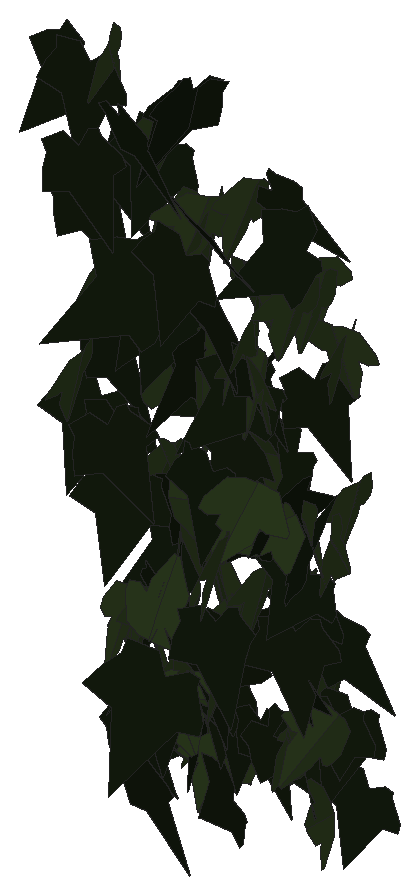
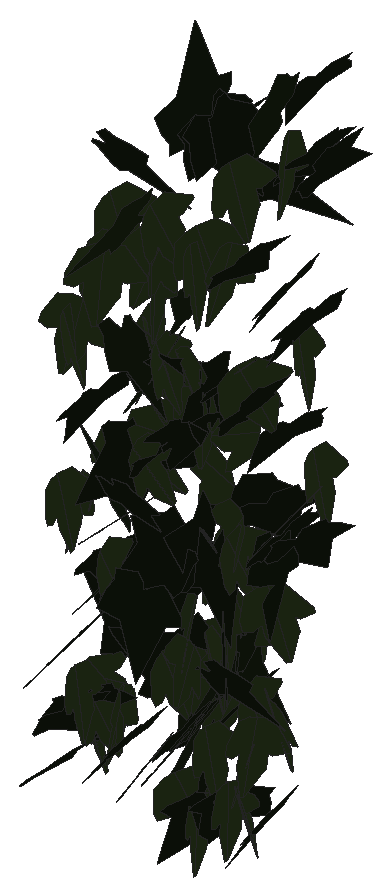
# SketchUp Ruby script. Lengths in inches.
U = 1.inch
M = Sketchup.active_model
def pt(a) = Geom::Point3d.new(a.map { |v| v * U })
def face(e, loops, mat)
  f = e.add_face(loops[0].map { |a| pt(a) })
  loops[1..].each { |l| e.add_face(l.map { |a| pt(a) }).erase! }
  f.material = f.back_material = mat if mat
  f
end
# faces: each face lists its corners as indices into pts; further lists are holes
def faces(e, pts, list, mat = nil) = list.each { |f| face(e, (f[0].is_a?(Array) ? f : [f]).map { |l| l.map { |i| pts[i] } }, mat) }
# xy, xz, yz: faces in a plane at the given z, y or x. An outline is a flat list of corners, or four numbers for a rectangle; further outlines are holes
def ring(l) = l.size == 4 ? [[l[0], l[1]], [l[2], l[1]], [l[2], l[3]], [l[0], l[3]]] : l.each_slice(2).to_a
def flat(e, list, mat, &to3) = list.each { |f| face(e, (f[0].is_a?(Array) ? f : [f]).map { |l| ring(l).map { |u, v| to3.(u, v) } }, mat) }
def xy(e, z, list, mat = nil) = flat(e, list, mat) { |x, y| [x, y, z] }
def xz(e, y, list, mat = nil) = flat(e, list, mat) { |x, z| [x, y, z] }
def yz(e, x, list, mat = nil) = flat(e, list, mat) { |y, z| [x, y, z] }
def lines(e, pts, list) = list.each { |a, b| e.add_line(pt(pts[a]), pt(pts[b])) }
# prism: a flat outline (further loops are holes) pulled along v
def prism(e, loops, v, mat = nil)
  f = face(e, loops, mat); d = Geom::Vector3d.new(v.map { |x| x * U })
  f.pushpull(f.normal.samedirection?(d) ? d.length : -d.length)
end
def box(e, o, s, mat = nil) = prism(e, [[o, [o[0] + s[0], o[1], o[2]], [o[0] + s[0], o[1] + s[1], o[2]], [o[0], o[1] + s[1], o[2]]]], [0, 0, s[2]], mat)
def at(x, y, z, deg = 0) = Geom::Transformation.translation(pt([x, y, z])) * Geom::Transformation.rotation(ORIGIN, Z_AXIS, deg.degrees)
def axes(o, x, y, z) = Geom::Transformation.new([*x, 0, *y, 0, *z, 0, *pt(o).to_a, 1])
def part(name) = M.definitions.add(name)
# library, detail: a bought-in or finely detailed component or shape, given as its bounding box
def library(name, o, s) = part(name).tap { |d| box(d.entities, o, s) }
def detail(e, o, s) = box(e.add_group.entities, o, s)
def put(e, d, t, mat = nil) = e.add_instance(d, t).tap { |i| i.material = mat if mat }
def group(e, t, mat = nil) = e.add_group.tap { |g| g.transformation = t; g.material = mat if mat }.entities
root = M.entities
M.materials.add("efeu1").color = [18, 25, 13]
M.materials.add("efeu2").color = [43, 57, 29]
c1 = part("ivyleaf_9")
p = [[1.54,2.16,1.25],[1.36,2.04,1.19],[-0.21,0.99,0.68],[-0.71,1.11,0.82],[-0.85,0.86,0.67],[-0.8,0.17,0.21],
  [-0.9,-0.01,0.1],[-0.67,-0.16,-0.02],[-0.08,-0.08,-0.05],[-0.03,-0.6,-0.4],[0.65,-0.88,-0.66],[0.83,-0.6,-0.49],
  [1.29,-0.42,-0.43],[1.8125,-0.07,-0.26],[1.21,0.44,0.15]]
faces(c1.entities,p,[[0,1,2,3,4,5,6,7,8,9,10,11,12,13,14]],"efeu1")
c2 = part("ivyleaf_10")
p = [[0,0.5,-0.03],[-0.0625,2.02,-0.43],[-0.19,2.01,-0.46],[-0.54,1.05,-0.29],[-0.52,0.625,-0.18],[-0.83,0.76,-0.28],
  [-1.16,0.64,-0.33],[-1.15,0.33,-0.24],[-0.77,-0.39,0.02],[-0.3,-0.51,0.16],[0.04,-0.48,0.23],[-0.02,2.01,-0.4375],
  [-0.06,2.01,-0.43],[0.04,-0.49,0.23],[0.67,-0.49,0.14],[1.38,0.36,-0.2],[1.375,0.51,-0.24],[0.81,0.65,-0.19],
  [0.62,0.59,-0.15],[0.6,1.09,-0.28],[0.5,1.23,-0.31]]
faces(c2.entities,p,[[0,1,2,3,4,5,6,7,8,9,10],[11,12,0,13,14,15,16,17,18,19,20]],"efeu2")
put(root,c1,axes([550.52,126.8,290.29],[0.5719,-0.99368,-0.26786],[-0.00484,0.30384,-1.13749],[1.02914,0.55363,0.1435]))
put(root,c1,axes([551.15,125.6875,288.58],[-0.4997,-1.07408,0.06515],[-0.00721,-0.06848,-1.18442],[1.07603,-0.49925,0.02231]))
put(root,c2,axes([551.51,124.1,290.82],[0.18064,-1.20547,-0.05667],[-0.00234,0.05695,-1.21892],[1.2068,0.18055,0.00612]))
put(root,c2,axes([551.94,126.33,285.9375],[-1.04432,-0.39407,0.41704],[-0.30298,-0.35673,-1.0958],[0.48725,-1.06643,0.21245]))
put(root,c1,axes([551.4,124.52,297.51],[0.44186,-1.01629,-0.53112],[-0.03486,0.55702,-1.09484],[1.14617,0.40873,0.17145]))
put(root,c1,axes([551.97,123.53,302.78],[-0.34838,-0.90881,0.76609],[-0.28525,-0.71107,-0.97325],[1.15389,-0.45017,-0.00929]))
put(root,c2,axes([552.04,127.11,280.74],[-0.36388,-1.02386,-0.3654],[0.14113,0.33758,-1.08643],[1.07791,-0.38983,0.0189]))
put(root,c1,axes([552.49,125.39,287.5625],[0.62271,0.33075,-0.97016],[-1.01556,0.04545,-0.63636],[-0.13873,1.15192,0.30367]))
put(root,c2,axes([552.21,125.68,280.95],[0.98533,-0.69641,-0.01824],[-0.02055,0.00252,-1.20655],[0.69634,0.98549,-0.0098]))
put(root,c1,axes([551.92,125.27,298.84],[0.52048,-1.05811,-0.30369],[-0.04902,0.31331,-1.17565],[1.09973,0.51474,0.09133]))
put(root,c1,axes([552.2,125.37,288.23],[0.10674,-1.18347,-0.07002],[-0.01361,0.06907,-1.18825],[1.18546,0.10735,-0.00734]))
put(root,c2,axes([552.875,123.34,295.21],[0.35374,-1.15693,-0.2481],[-0.0681,0.23861,-1.20979],[1.18127,0.36021,0.00455]))
put(root,c2,axes([552.6875,126.8125,279.45],[-0.66655,0.95154,-0.11806],[0.08029,-0.08788,-1.16168],[-0.95547,-0.67119,-0.01526]))
put(root,c1,axes([552.375,125.69,276.73],[0.61516,-0.84906,-0.46175],[-0.15079,0.45633,-1.03999],[0.95466,0.61919,0.13328]))
put(root,c2,axes([552.83,126.88,277.54],[0.71382,-0.89446,0.08275],[0.04138,-0.07284,-1.14431],[0.89733,0.7149,-0.01306]))
put(root,c1,axes([553.51,127.61,282.9375],[-1.1354,0.01597,0.18946],[-0.18921,0.01832,-1.13541],[-0.01877,-1.15095,-0.01544]))
put(root,c2,axes([552.97,127.43,277.84],[0.01512,-1.1208,-0.20504],[0.11901,0.20549,-1.11448],[1.13316,-0.00662,0.11978]))
put(root,c1,axes([552.63,123.28,303.125],[-0.09536,-1.22202,0.15335],[0.01995,-0.15533,-1.22532],[1.23144,-0.09211,0.03173]))
put(root,c2,axes([553,123.875,303.47],[0.31117,-1.09953,-0.51575],[0.09795,0.55339,-1.12069],[1.21052,0.23786,0.22325]))
put(root,c2,axes([553.05,126.02,281.24],[0.13344,-1.06932,0.45628],[0.17655,-0.43532,-1.07181],[1.14912,0.19105,0.11169]))
put(root,c1,axes([553.51,126.07,293.33],[-0.35755,-0.99389,0.54034],[-0.12738,-0.52771,-1.05495],[1.12408,-0.37594,0.05232]))
put(root,c1,axes([553.26,126.71,277.49],[0.02789,-0.87016,-0.75638],[0.12703,0.75431,-0.8631],[1.14593,-0.06244,0.11409]))
put(root,c2,axes([554.02,125.23,294.02],[-0.63948,-0.84249,0.57455],[-0.16374,-0.58454,-1.03939],[1.00652,-0.63036,0.19594]))
put(root,c2,axes([553.86,125.98,287.23],[0.11183,-1.10768,0.4077],[0.01612,-0.40806,-1.11307],[1.18022,0.11053,-0.02343]))
put(root,c1,axes([554.5,125.94,283.7],[-0.09017,0.24721,-1.19825],[-1.17132,0.32966,0.15615],[0.35345,1.15553,0.2118]))
put(root,c1,axes([553.9,125.85,299.1875],[-0.3624,-1.09574,0.35859],[-0.00054,-0.37572,-1.14865],[1.15292,-0.34461,0.11218]))
put(root,c2,axes([554.24,127.04,279.55],[0.02016,-1.1673,-0.03753],[-0.00817,0.03739,-1.16745],[1.16787,0.02042,-0.00752]))
put(root,c1,axes([554.75,124.21,281.6875],[-0.82438,0.49475,-0.73156],[0.57258,-0.4625,-0.95802],[-0.67239,-1.00044,0.08111]))
put(root,c2,axes([554.69,124.25,291.16],[0.22597,-0.48447,1.12183],[-0.35131,1.06693,0.53152],[-1.17039,-0.41379,0.05705]))
put(root,c1,axes([554.14,127.22,277.04],[0.00901,-0.68641,-0.91145],[0.1707,0.90203,-0.67763],[1.12817,-0.131,0.10981]))
put(root,c2,axes([554.6875,127.1,276.56],[0.15834,-1.07209,-0.37597],[0.03088,0.38352,-1.08062],[1.13568,0.13904,0.0818]))
put(root,c2,axes([554.91,125.05,283.91],[0.32838,-0.97487,-0.56849],[-0.13018,0.55539,-1.0276],[1.12098,0.35008,0.0472]))
put(root,c1,axes([554.68,123.04,287.63],[-0.52217,-1.08101,-0.06386],[0.0193,0.06159,-1.20048],[1.08272,-0.52244,-0.0094]))
put(root,c2,axes([554.5,125.32,287.78],[-0.86964,0.69627,-0.46587],[0.39264,-0.25442,-1.1132],[-0.74004,-0.9532,-0.04317]))
put(root,c1,axes([554.18,125.51,281.9375],[0.21494,-0.76707,0.87556],[0.30031,-0.82368,-0.79534],[1.12464,0.36654,0.04504]))
put(root,c1,axes([554.28,126.39,281.03],[0.45392,-1.08437,0.1036],[0.04129,-0.09503,-1.17554],[1.08852,0.45579,0.00138]))
put(root,c1,axes([555.45,125.24,286.47],[0.6219,0.35974,-1.02332],[-0.96771,-0.3489,-0.71075],[-0.49004,1.14552,0.10489]))
put(root,c1,axes([554.84,125.01,293.68],[-0.3392,-1.08928,0.3941],[0.0689,-0.4289,-1.12614],[1.15633,-0.29397,0.18271]))
put(root,c2,axes([555.24,124.3,301.6],[-0.20561,-1.21741,0.16391],[-0.00308,-0.16567,-1.23441],[1.22839,-0.20419,0.02434]))
put(root,c2,axes([555.16,127.16,282.84],[-1.02059,0.51251,-0.21088],[0.1211,-0.22499,-1.13289],[-0.54081,-1.01757,0.14428]))
put(root,c1,axes([554.7,121.82,290.4],[0.23011,-1.06456,-0.52231],[0.13233,0.55179,-1.06633],[1.17838,0.14592,0.22174]))
put(root,c2,axes([555.5625,125.26,282.26],[0.54549,-1.03915,-0.18769],[-0.0893,0.1651,-1.17362],[1.05218,0.55275,-0.0023]))
put(root,c2,axes([555.23,123.63,282.28],[1.17243,0.25903,-0.33483],[0.32687,0.0726,1.2007],[0.26901,-1.21714,0.00036]))
put(root,c1,axes([555.09,126.26,278],[-0.00023,-0.08305,-1.23674],[1.09317,-0.58301,0.03894],[-0.58431,-1.0907,0.07335]))
put(root,c1,axes([555.17,124.03,279.59],[0.11854,-1.13736,0.27835],[0.08048,-0.2712,-1.14241],[1.16816,0.1341,0.05046]))
put(root,c2,axes([555.65,124.11,297.98],[-0.02558,-1.09118,-0.55827],[0.27972,0.53845,-1.06527],[1.19335,-0.14961,0.23773]))
put(root,c2,axes([556.01,125.93,283.94],[-0.75738,0.80985,0.30465],[-0.25376,0.17917,-1.10716],[-0.82721,-0.79645,0.06071]))
put(root,c2,axes([555.78,122.27,280.27],[0.70255,-0.9017,0.30657],[0.18777,-0.24234,-1.14308],[0.9337,0.72721,-0.00079]))
put(root,c2,axes([555.73,123.78,279.71],[0.5871,0.98322,0.40408],[0.19554,0.35385,-1.14509],[-1.04487,0.61868,0.01276]))
put(root,c2,axes([556.26,124.72,280.59],[0.02201,0.66275,-1.06763],[-0.36783,-1.01762,-0.6393],[-1.20157,0.32365,0.17615]))
put(root,c2,axes([556.36,126.07,276.56],[-0.72027,-0.72825,0.49988],[-0.07978,-0.58873,-0.97265],[0.87969,-0.64966,0.32108]))
put(root,c1,axes([556.36,124.85,285.95],[-0.05705,-0.05588,1.254],[0.42166,1.1815,0.07183],[-1.18231,0.42406,-0.03489]))
put(root,c2,axes([556.41,126.67,281.84],[-0.11059,-1.09252,0.37054],[0.04543,-0.37607,-1.09528],[1.15275,-0.09,0.07871]))
put(root,c1,axes([555.96,126.4,279.25],[0.06172,-1.14293,0.20643],[0.01395,-0.20597,-1.14459],[1.16134,0.06321,0.00278]))
put(root,c1,axes([555.65,121.3,302.91],[0.95773,-0.91663,0.09489],[0.08147,-0.0521,-1.32556],[0.91792,0.961,0.01864]))
put(root,c1,axes([556.37,124.74,292.61],[-0.19347,0.04003,-1.17983],[0.66689,-0.98281,-0.14271],[-0.97409,-0.68082,0.13663]))
put(root,c1,axes([555.79,125.84,279.5625],[0.3529,-0.95674,0.57398],[0.23817,-0.52353,-1.01909],[1.08999,0.42415,0.03685]))
put(root,c1,axes([556.71,123.68,303.19],[-0.17396,0.73755,-1.01767],[0.2869,-0.97694,-0.75708],[-1.22365,-0.33391,-0.03283]))
put(root,c2,axes([556.73,124.34,298.47],[-0.61435,-0.99369,0.40384],[-0.07888,-0.42228,-1.15905],[1.06971,-0.60183,0.14647]))
put(root,c2,axes([556.57,125.03,297.97],[0.28832,-1.16287,-0.21213],[0.01604,0.22217,-1.19615],[1.18195,0.28065,0.06798]))
put(root,c2,axes([555.68,125.05,285.56],[-0.09914,0.01628,-1.24758],[0.9745,-0.78052,-0.08762],[-0.77914,-0.9783,0.04915]))
put(root,c1,axes([556,118.6,303.09],[0.25925,-1.17083,-0.34469],[0.03767,0.35989,-1.19412],[1.21993,0.2377,0.11012]))
put(root,c1,axes([556.77,123.64,303.3],[-0.31673,0.63119,-1.05487],[0.45358,-0.95246,-0.7061],[-1.14255,-0.55308,0.01211]))
put(root,c2,axes([556.89,124.31,291.58],[-1.14621,0.3522,0.17655],[-0.22743,-0.14802,-1.18126],[-0.3217,-1.15024,0.20607]))
put(root,c1,axes([556.33,125.46,291.46],[-0.1502,-1.08353,-0.52219],[0.23482,0.4897,-1.08367],[1.17965,-0.23544,0.14923]))
put(root,c1,axes([557.13,127.15,284.85],[0.19985,1.1489,0.00557],[-0.03076,0.011,-1.16571],[-1.1485,0.19962,0.03219]))
put(root,c1,axes([556.52,126.53,278.06],[0.12882,-1.07402,0.41956],[0.08882,-0.41167,-1.0811],[1.14964,0.15216,0.03651]))
put(root,c2,axes([557.53,124.28,293],[0.74055,-0.58601,-0.82168],[-0.62429,0.53479,-0.94405],[0.79299,0.96828,0.02413]))
put(root,c1,axes([556.58,126.1,286.53],[1.16067,0.13063,0.24963],[0.25235,-0.01145,-1.16736],[-0.12529,1.18716,-0.03873]))
put(root,c2,axes([557.3,125.21,281.02],[0.33325,-0.98199,0.59413],[0.216,-0.55396,-1.03675],[1.12723,0.39646,0.02301]))
put(root,c1,axes([557.05,124.89,280.72],[-0.16149,-0.03357,1.25588],[1.1624,0.47642,0.1622],[-0.47666,1.17318,-0.02993]))
put(root,c1,axes([558.47,119.2,298.41],[-1.34669,-0.23569,0.48348],[-0.46918,-0.1226,-1.36664],[0.263,-1.42559,0.0376]))
put(root,c1,axes([557.24,126.9,277.5625],[0.48637,-1.04803,-0.04095],[-0.01585,0.03778,-1.15538],[1.04871,0.48662,0.00152]))
put(root,c2,axes([556.97,123.04,288.01],[0.28249,-0.11424,-1.22465],[1.11812,-0.49967,0.30453],[-0.51245,-1.15321,-0.01063]))
put(root,c2,axes([558.63,125.38,289.21],[0.47294,0.02208,-1.06905],[-0.89836,0.64218,-0.38417],[0.57992,0.97681,0.27673]))
put(root,c1,axes([557.88,125.44,289.66],[-0.50357,-1.04626,0.29042],[-0.03977,-0.30215,-1.15746],[1.08509,-0.49662,0.09236]))
put(root,c1,axes([557.83,124.52,275.87],[-0.27081,-0.4097,1.04657],[0.02093,-1.07817,-0.41666],[1.12371,-0.07865,0.25998]))
put(root,c2,axes([558.18,124.81,293.33],[0.24935,-1.14895,0.25092],[0.06378,-0.24291,-1.17565],[1.1743,0.25716,0.01057]))
put(root,c2,axes([558.18,125.08,299.26],[-0.01835,-1.08463,0.54593],[0.13514,-0.54442,-1.0771],[1.20673,0.04447,0.12892]))
put(root,c2,axes([558.31,125.62,284.23],[0.03834,-1.17333,0.0616],[-0.00774,-0.06189,-1.17392],[1.17492,0.03788,-0.00974]))
put(root,c1,axes([558.65,126.88,288.56],[-1.16457,-0.061,-0.17261],[0.17281,0.00067,-1.16614],[0.06044,-1.1773,0.00828]))
put(root,c1,axes([557.67,123.47,295.5],[0.53065,-0.99909,0.44125],[0.19677,-0.39509,-1.13122],[1.07432,0.56585,-0.01076]))
put(root,c1,axes([558.95,124.49,292.33],[-1.01158,-0.58175,0.34738],[-0.29863,-0.17751,-1.16692],[0.60821,-1.05473,0.00479]))
put(root,c1,axes([558.22,123.17,283.38],[0.01377,-1.18213,-0.28498],[0.04374,0.2853,-1.18133],[1.21521,0.00312,0.04575]))
put(root,c1,axes([558.23,124.77,293.15],[0.71223,-0.94681,-0.23207],[-0.15833,0.17125,-1.18456],[0.9619,0.72925,-0.02314]))
put(root,c1,axes([558.0625,119.32,279.32],[0.82891,-1.0411,0.02855],[0.01508,-0.02449,-1.33078],[1.04138,0.82904,-0.00346]))
put(root,c1,axes([558.52,122.6,289.57],[-0.01734,-1.15,0.38369],[0.04714,-0.38408,-1.14904],[1.2114,-0.00151,0.0502]))
put(root,c1,axes([558.43,125.91,278.1875],[0.63497,-0.82265,-0.53617],[-0.07442,0.59634,-1.00312],[0.97913,0.57882,0.27146]))
put(root,c1,axes([559.6,125.34,294.0625],[-0.67441,0.99577,-0.21635],[0.06386,-0.21764,-1.20073],[-1.017,-0.67399,0.06808]))
put(root,c2,axes([559.27,123.92,297.03],[-1.19159,0.27243,-0.25757],[0.25439,-0.04291,-1.22225],[-0.2754,-1.21835,-0.01455]))
put(root,c2,axes([559.26,124.125,293.27],[0.94444,-0.74722,0.2022],[0.16639,-0.11555,-1.20422],[0.756,0.9589,0.01245]))
put(root,c1,axes([558.87,125.64,299.3],[0.98924,-0.57074,-0.41456],[-0.15431,0.52166,-1.0864],[0.68833,0.93719,0.35225]))
put(root,c2,axes([559.55,123.56,293.59],[-0.99194,0.74992,0.06036],[-0.05263,0.03047,-1.24349],[-0.7505,-0.99331,0.00742]))
put(root,c2,axes([559.69,123.25,295.67],[0.26942,-1.02488,-0.67232],[-0.12172,0.66259,-1.05883],[1.21966,0.29252,0.04284]))
put(root,c2,axes([559.85,127.65,280.43],[0.12463,-1.12383,-0.13995],[0.00156,0.14097,-1.1306],[1.13251,0.12348,0.01696]))
put(root,c2,axes([559.78,125.13,278.47],[0.24985,-0.9244,-0.61852],[0.11262,0.6517,-0.92849],[1.10652,0.1424,0.23416]))
put(root,c2,axes([560.06,126.34,278.85],[-0.03055,-1.09356,0.41182],[-0.01198,-0.41165,-1.09399],[1.16848,-0.03281,-0.00045]))
put(root,c1,axes([560.07,117.92,284.18],[-1.10727,-0.93895,-0.17797],[0.12879,0.12329,-1.45175],[0.94695,-1.11468,-0.01065]))
put(root,c2,axes([560.66,123.51,288.11],[0.75213,0.01163,-0.98265],[-0.98237,-0.02391,-0.7522],[-0.02605,1.23723,-0.0053]))
put(root,c2,axes([560.17,122.5,289.26],[0.96145,0.62706,-0.49269],[-0.41187,-0.27039,-1.14786],[-0.68287,1.04596,-0.00136]))
put(root,c2,axes([560.04,125.73,284.4375],[0.27838,-1.05246,0.46755],[0.1924,-0.43175,-1.08643],[1.13545,0.3312,0.06946]))
put(root,c1,axes([559.8125,119.46,299.82],[-0.18778,-1.13105,0.46989],[0.06317,-0.48369,-1.13902],[1.22314,-0.14866,0.13096]))
put(root,c2,axes([560.43,125.54,296.9],[-0.87558,-0.81148,-0.09942],[0.05387,0.0881,-1.19346],[0.81577,-0.87679,-0.0279]))
put(root,c1,axes([559.96,126.15,283.67],[-0.0423,-1.07311,0.48491],[0.15869,-0.48599,-1.06166],[1.16684,0.02719,0.16196]))
put(root,c1,axes([560.55,123.55,288.14],[-0.22783,0.41966,-1.141],[-0.52855,1.01122,0.47746],[1.09482,0.57552,-0.00693]))
put(root,c1,axes([560,126.37,291.97],[0.29087,-1.07246,-0.43117],[-0.02372,0.43898,-1.10789],[1.15565,0.27894,0.08578]))
put(root,c2,axes([560.51,120.52,288.23],[0.50332,-1.06163,0.34009],[0.15862,-0.30114,-1.17482],[1.10343,0.52754,0.01376]))
put(root,c1,axes([560.57,126.66,279],[-0.53831,-1.01708,-0.1947],[0.07661,0.17972,-1.15064],[1.03271,-0.5435,-0.01613]))
put(root,c2,axes([560.94,125.73,279.23],[-0.35737,-0.69954,0.92647],[-0.03446,-0.96255,-0.74008],[1.16039,-0.24402,0.26334]))
put(root,c1,axes([560.3,127.03,281.99],[0.6938,-0.80727,-0.48232],[-0.09641,0.53516,-1.0344],[0.93543,0.6539,0.25112]))
put(root,c1,axes([560.7,127.41,278.8],[-0.37721,-1.08245,0.13515],[-0.00116,-0.1426,-1.14539],[1.09085,-0.37446,0.04551]))
put(root,c1,axes([560.73,125.04,285.4],[-0.47345,-0.9157,0.59609],[0.0987,-0.68283,-0.97056],[1.08816,-0.33648,0.34739]))
put(root,c2,axes([561.05,127.11,287.78],[-0.00319,-1.1655,0.03473],[0.00056,-0.03473,-1.16551],[1.16602,-0.00317,0.00066]))
put(root,c1,axes([560.06,124.6,281.92],[0.66398,-0.12698,-1.09291],[1.10019,0.06232,0.66117],[-0.01233,-1.27728,0.14091]))
put(root,c2,axes([561.08,125.15,296.73],[-0.01215,-1.12219,0.41483],[0.16592,-0.41243,-1.11082],[1.18485,0.04625,0.15981]))
put(root,c1,axes([560.35,120.06,300.47],[1.25493,-0.45203,-0.48301],[0.45294,-0.16782,1.33385],[-0.48216,-1.33416,-0.00413]))
put(root,c1,axes([561.02,123.78,285.96],[-0.3707,1.0118,0.57922],[0.17495,-0.55264,1.07734],[1.15267,0.40928,0.02277]))
put(root,c2,axes([561.4,126.23,294.125],[0.38503,-1.13199,0.04812],[0.00705,-0.04843,-1.19564],[1.13299,0.38499,-0.00891]))
put(root,c2,axes([561.42,125.85,294.5],[-1.19569,0.01771,-0.08918],[0.08872,-0.03049,-1.19547],[-0.01992,-1.19863,0.02909]))
put(root,c1,axes([561.21,123.77,283.79],[-0.14994,-1.13905,-0.28751],[0.08834,0.27809,-1.1478],[1.17145,-0.16676,0.04976]))
put(root,c2,axes([561.64,125.1875,286.81],[0.33391,-0.86688,-0.74676],[0.03725,0.78574,-0.89547],[1.14357,0.22753,0.24722]))
put(root,c2,axes([561.74,123.86,288.01],[-0.76911,0.90288,0.31585],[-0.20536,0.23998,-1.18605],[-0.93423,-0.79605,0.00069]))
put(root,c2,axes([562.13,124.21,276.89],[0.59565,-0.50535,-0.9431],[-0.62692,0.70986,-0.77632],[0.86705,0.86042,0.08657]))
put(root,c2,axes([561.82,123.03,297.52],[-0.15679,-1.22936,0.23126],[0.01145,-0.23447,-1.23866],[1.25087,-0.15194,0.04032]))
put(root,c1,axes([562.46,122.52,299.66],[-1.22656,0.13213,0.29706],[-0.29429,0.04156,-1.23362],[-0.13818,-1.26134,-0.00953]))
put(root,c1,axes([561.41,127.39,276.23],[-0.29394,-1.03678,0.40255],[0.14553,-0.44865,-1.04923],[1.10262,-0.21717,0.2458]))
